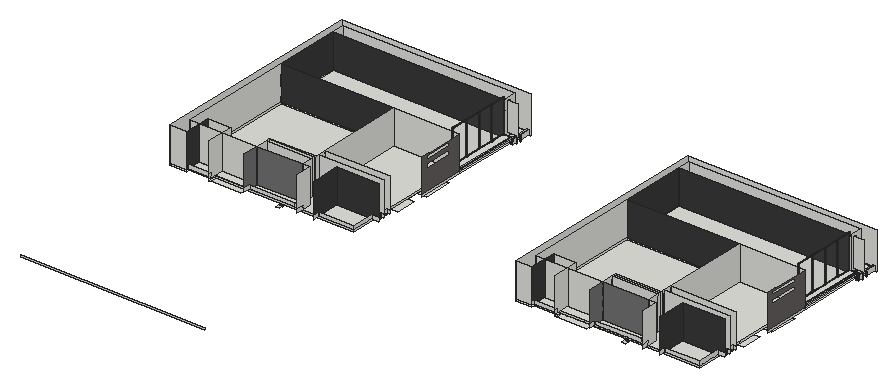
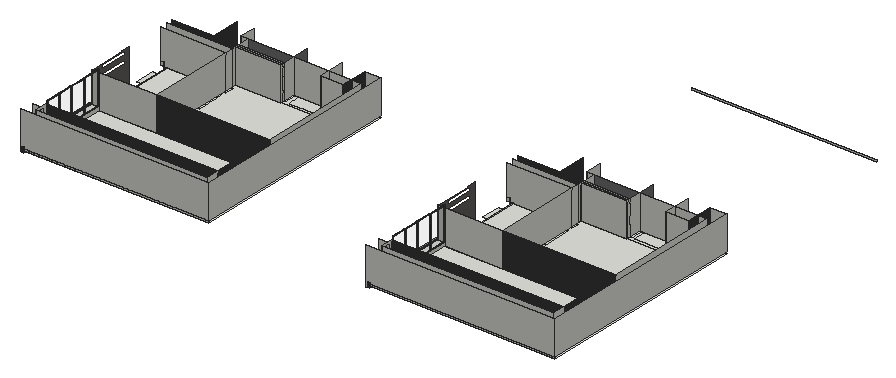
# SketchUp Ruby script. Lengths in inches.
U = 1.inch
M = Sketchup.active_model
def pt(a) = Geom::Point3d.new(a.map { |v| v * U })
def face(e, loops, mat)
  f = e.add_face(loops[0].map { |a| pt(a) })
  loops[1..].each { |l| e.add_face(l.map { |a| pt(a) }).erase! }
  f.material = f.back_material = mat if mat
  f
end
# faces: each face lists its corners as indices into pts; further lists are holes
def faces(e, pts, list, mat = nil) = list.each { |f| face(e, (f[0].is_a?(Array) ? f : [f]).map { |l| l.map { |i| pts[i] } }, mat) }
# xy, xz, yz: faces in a plane at the given z, y or x. An outline is a flat list of corners, or four numbers for a rectangle; further outlines are holes
def ring(l) = l.size == 4 ? [[l[0], l[1]], [l[2], l[1]], [l[2], l[3]], [l[0], l[3]]] : l.each_slice(2).to_a
def flat(e, list, mat, &to3) = list.each { |f| face(e, (f[0].is_a?(Array) ? f : [f]).map { |l| ring(l).map { |u, v| to3.(u, v) } }, mat) }
def xy(e, z, list, mat = nil) = flat(e, list, mat) { |x, y| [x, y, z] }
def xz(e, y, list, mat = nil) = flat(e, list, mat) { |x, z| [x, y, z] }
def yz(e, x, list, mat = nil) = flat(e, list, mat) { |y, z| [x, y, z] }
def lines(e, pts, list) = list.each { |a, b| e.add_line(pt(pts[a]), pt(pts[b])) }
# prism: a flat outline (further loops are holes) pulled along v
def prism(e, loops, v, mat = nil)
  f = face(e, loops, mat); d = Geom::Vector3d.new(v.map { |x| x * U })
  f.pushpull(f.normal.samedirection?(d) ? d.length : -d.length)
end
def box(e, o, s, mat = nil) = prism(e, [[o, [o[0] + s[0], o[1], o[2]], [o[0] + s[0], o[1] + s[1], o[2]], [o[0], o[1] + s[1], o[2]]]], [0, 0, s[2]], mat)
def at(x, y, z, deg = 0) = Geom::Transformation.translation(pt([x, y, z])) * Geom::Transformation.rotation(ORIGIN, Z_AXIS, deg.degrees)
def axes(o, x, y, z) = Geom::Transformation.new([*x, 0, *y, 0, *z, 0, *pt(o).to_a, 1])
def part(name) = M.definitions.add(name)
# library, detail: a bought-in or finely detailed component or shape, given as its bounding box
def library(name, o, s) = part(name).tap { |d| box(d.entities, o, s) }
def detail(e, o, s) = box(e.add_group.entities, o, s)
def put(e, d, t, mat = nil) = e.add_instance(d, t).tap { |i| i.material = mat if mat }
def group(e, t, mat = nil) = e.add_group.tap { |g| g.transformation = t; g.material = mat if mat }.entities
root = M.entities
M.materials.add("Glazing").color = [128, 128, 128]
M.materials["Glazing"].alpha = 0.05
M.materials.add("Powdercoating").color = [41, 44, 40]
M.materials.add("[Color M05]").color = [114, 114, 114]
M.materials.add("[Color M07]").color = [58, 58, 58]
M.materials.add("[Concrete Tile]").color = [165, 155, 133]
M.materials.add("[Stone Marble]").color = [99, 95, 94]
c1 = part("Group\#15")
xy(c1.entities,0,[[0,-55.94,0.71,45.94]])
xy(c1.entities,0.2,[[0,-55.94,0.47,45.94],[0.47,45.94,0.71,46.42]])
xy(c1.entities,2.36,[[0.47,-55.94,0.71,46.42]])
xz(c1.entities,-55.94,[[0,0,0.71,0,0.71,2.36,0.47,2.36,0.47,0.2,0,0.2]])
xz(c1.entities,45.94,[[0,0,0.71,0.2]])
xz(c1.entities,46.42,[[0.47,0.2,0.71,2.36]])
yz(c1.entities,0,[[-55.94,0,45.94,0.2]])
yz(c1.entities,0.47,[[-55.94,0.2,46.42,2.36]])
yz(c1.entities,0.71,[[-55.94,0,45.94,0,45.94,0.2,46.42,0.2,46.42,2.36,-55.94,2.36]])
c2 = part("Group\#7")
xy(c2.entities,0,[[0,-59.09,0.71,45.94]])
xy(c2.entities,0.2,[[0,-59.09,0.47,45.94],[0.47,45.94,0.71,46.42]])
xy(c2.entities,2.36,[[0.47,-59.09,0.71,46.42]])
xz(c2.entities,-59.09,[[0,0,0.71,0,0.71,2.36,0.47,2.36,0.47,0.2,0,0.2]])
xz(c2.entities,45.94,[[0,0,0.71,0.2]])
xz(c2.entities,46.42,[[0.47,0.2,0.71,2.36]])
yz(c2.entities,0,[[-59.09,0,45.94,0.2]])
yz(c2.entities,0.47,[[-59.09,0.2,46.42,2.36]])
yz(c2.entities,0.71,[[-59.09,0,45.94,0,45.94,0.2,46.42,0.2,46.42,2.36,-59.09,2.36]])
c3 = part("Group\#16")
prism(c3.entities,[[[0.47,-56.18,0.2],[0,-56.18,0.2],[0,-56.18,0],[0.71,-56.18,0],[0.71,-56.18,2.36],[0.47,-56.18,2.36]]],[0,28.68,0])
c4 = part("Group\#10")
box(c4.entities,[-0.73,0,0],[27.99,0.55,102.05])
c5 = part("Group\#18")
xy(c5.entities,0,[[0.47,-56.18,0.47,-55.47,0,-55.47,0,-28.21,1.18,-28.21,1.18,-56.18]])
xy(c5.entities,0.2,[[0.71,-56.18,1.18,-28.21],[0,-55.47,0.47,-28.21],[0.47,-28.21,0.71,-27.74]])
xy(c5.entities,2.36,[[0.47,-56.18,0.71,-27.74]])
xz(c5.entities,-56.18,[[0.47,0,1.18,0,1.18,0.2,0.71,0.2,0.71,2.36,0.47,2.36]])
xz(c5.entities,-55.47,[[0,0,0.47,0.2]])
xz(c5.entities,-28.21,[[0,0,1.18,0.2]])
xz(c5.entities,-27.74,[[0.47,0.2,0.71,2.36]])
yz(c5.entities,0,[[-55.47,0,-28.21,0.2]])
yz(c5.entities,0.47,[[-56.18,0,-55.47,0.2],[-56.18,0.2,-27.74,2.36]])
yz(c5.entities,0.71,[[-56.18,0.2,-27.74,2.36]])
yz(c5.entities,1.18,[[-56.18,0,-28.21,0.2]])
c6 = part("Group\#34")
xy(c6.entities,0,[[-20.45,0,7.76,1.22]])
xy(c6.entities,0.06,[[-20.39,0.06,7.7,1.22]])
xy(c6.entities,0.47,[[-19.98,0,7.28,0.06]])
xy(c6.entities,101.89,[[-19.98,0,7.28,0.06]])
xy(c6.entities,102.3,[[-20.39,0.06,7.7,1.22]])
xy(c6.entities,102.36,[[-20.45,0,7.76,1.22]])
xz(c6.entities,0,[[[-20.45,0,7.76,102.36],[-19.98,0.47,7.28,101.89]]])
xz(c6.entities,0.06,[[[-20.39,0.06,7.7,102.3],[-19.98,0.47,7.28,101.89]]])
xz(c6.entities,1.22,[[[-20.45,0,7.76,102.36],[-20.39,0.06,7.7,102.3]]])
yz(c6.entities,-20.45,[[0,0,1.22,102.36]])
yz(c6.entities,-20.39,[[0.06,0.06,1.22,102.3]])
yz(c6.entities,-19.98,[[0,0.47,0.06,101.89]])
yz(c6.entities,7.28,[[0,0.47,0.06,101.89]])
yz(c6.entities,7.7,[[0.06,0.06,1.22,102.3]])
yz(c6.entities,7.76,[[0,0,1.22,102.36]])
c7 = part("Group\#6")
put(c7.entities,c1,axes([27.97,0,7.875],[1,0,0],[0,0,-1],[0,1,0]),"Powdercoating")
put(c7.entities,c2,axes([0.71,0,6.8],[-1,0,0],[0,0,-0.97687],[0,1,0]),"Powdercoating")
put(c7.entities,c3,axes([-27.5,0,-38.07],[0,0,-1],[-1,0,0],[0,1,0]),"Powdercoating")
put(c7.entities,c4,at(1.12,0.35,-38.39),"Glazing")
put(c7.entities,c5,axes([-27.5,0,63.35],[0,0,1],[-1,0,0],[0,1,0]),"Powdercoating")
put(c7.entities,c6,at(20.6875,1.0625,-38.54),"Powdercoating")
c8 = part("Sliding door assembly")
put(c8.entities,c7,at(-1.18,4.5,38.86))
g1 = group(c8.entities,at(84.74,4.5,38.86))
put(g1,c1,axes([-27.97,0,7.875],[-1,0,0],[0,0,-1],[0,1,0]),"Powdercoating")
put(g1,c2,axes([-0.71,0,6.8],[1,0,0],[0,0,-0.97687],[0,1,0]),"Powdercoating")
put(g1,c3,axes([27.5,0,-38.07],[0,0,-1],[1,0,0],[0,1,0]),"Powdercoating")
put(g1,c4,axes([-1.12,0.35,-38.39],[-1,0,0],[0,1,0],[0,0,1]),"Glazing")
put(g1,c5,axes([27.5,0,63.35],[0,0,1],[1,0,0],[0,1,0]),"Powdercoating")
put(g1,c6,axes([-20.6875,1.0625,-38.54],[-1,0,0],[0,1,0],[0,0,1]),"Powdercoating")
g2 = group(c8.entities,at(56.0625,4.5,38.86))
put(g2,c1,axes([-27.97,0,7.875],[-1,0,0],[0,0,-1],[0,1,0]),"Powdercoating")
put(g2,c3,axes([27.5,0,-38.07],[0,0,-1],[1,0,0],[0,1,0]),"Powdercoating")
put(g2,c4,axes([-1.12,0.35,-38.39],[-1,0,0],[0,1,0],[0,0,1]),"Glazing")
put(g2,c5,axes([27.5,0,63.35],[0,0,1],[1,0,0],[0,1,0]),"Powdercoating")
put(g2,c6,axes([-20.6875,1.0625,-38.54],[-1,0,0],[0,1,0],[0,0,1]),"Powdercoating")
g3 = group(g2,at(-0.71,0,6.8),"Powdercoating")
xy(g3,-45.34,[[0.47,0.2,0.71,2.36]])
xy(g3,-44.88,[[0,0,0.71,0.2]])
xy(g3,57.73,[[0,0,0.71,0,0.71,2.36,0.47,2.36,0.47,0.2,0,0.2]])
xz(g3,0,[[0,-44.88,0.71,57.73]])
xz(g3,0.2,[[0.47,-45.34,0.71,-44.88],[0,-44.88,0.47,57.73]])
xz(g3,2.36,[[0.47,-45.34,0.71,57.73]])
yz(g3,0,[[0,-44.88,0.2,57.73]])
yz(g3,0.47,[[0.2,-45.34,2.36,57.73]])
yz(g3,0.71,[[0.2,-45.34,2.36,-45.34,2.36,57.73,0,57.73,0,-44.88,0.2,-44.88]])
put(c8.entities,c7,axes([-33.94,4.5,38.86],[1.14218,0,0],[0,1,0],[0,0,1]))
c9 = part("sliding door")
put(c9.entities,c8,at(0,-4.5,-0.08))
xy(root,117.41,[[671.25,3528.25,913.875,3628.31],[1889.4375,3528.25,2132.0625,3628.31]])
xy(root,126,[[262.875,3214.625,262.875,3969.0625,913.875,3969.0625,913.875,3897.9,890.875,3897.9,890.875,3946.0625,285.875,3946.0625,285.875,3237.625,319.53,3237.625,319.53,3214.625],[399.88,3214.625,406.68,3237.625],[406.68,3214.625,511.23,3237.625],[634.11,3214.625,647.8,3229.61],[1481.0625,3214.625,1481.0625,3969.0625,2132.0625,3969.0625,2132.0625,3897.9,2109.0625,3897.9,2109.0625,3946.0625,1504.0625,3946.0625,1504.0625,3237.625,1537.72,3237.625,1537.72,3214.625],
  [1618.07,3214.625,1624.87,3237.625],[1624.87,3214.625,1729.42,3237.625],[1852.3,3214.625,1865.99,3229.61],[319.53,3226.125,399.88,3237.625],[1537.72,3226.125,1618.07,3237.625],
  [285.875,3237.625,319.53,3248.75],[319.53,3237.625,399.88,3248.75],[399.88,3237.625,406.68,3248.75],[406.68,3237.625,511.23,3248.75],[511.23,3237.625,521.59,3248.75],
  [521.59,3237.625,634.11,3248.75],[634.11,3237.625,709.87,3248.75],[709.87,3237.625,767.19,3248.75],[767.19,3237.625,817,3248.75],[817,3237.625,890.875,3248.75],
  [1504.0625,3237.625,1537.72,3248.75],[1537.72,3237.625,1618.07,3248.75],[1618.07,3237.625,1624.87,3248.75],[1624.87,3237.625,1729.42,3248.75],[1729.42,3237.625,1739.78,3248.75],
  [1739.78,3237.625,1852.3,3248.75],[1852.3,3237.625,1928.05,3248.75],[1928.05,3237.625,1985.38,3248.75],[1985.38,3237.625,2035.1875,3248.75],[2035.1875,3237.625,2109.0625,3248.75],
  [285.875,3248.75,319.53,3248.75,319.53,3307.9375,399.88,3307.9375,399.88,3248.75,406.68,3248.75,406.68,3307.9375,511.23,3307.9375,511.23,3248.75,521.59,3248.75,521.59,3307.9375,709.87,3307.9375,709.87,3248.75,767.19,3248.75,767.19,3317.34,285.875,3317.34],[319.53,3248.75,399.88,3307.9375],[406.68,3248.75,511.23,3307.9375],[521.59,3248.75,634.11,3307.9375],[634.11,3248.75,709.87,3307.9375],
  [767.19,3248.75,817,3317.34],[817,3248.75,890.875,3317.34],[1504.0625,3248.75,1537.72,3248.75,1537.72,3307.9375,1618.07,3307.9375,1618.07,3248.75,1624.87,3248.75,1624.87,3307.9375,1729.42,3307.9375,1729.42,3248.75,1739.78,3248.75,1739.78,3307.9375,1928.05,3307.9375,1928.05,3248.75,1985.38,3248.75,1985.38,3317.34,1504.0625,3317.34],[1537.72,3248.75,1618.07,3307.9375],[1624.87,3248.75,1729.42,3307.9375],
  [1739.78,3248.75,1852.3,3307.9375],[1852.3,3248.75,1928.05,3307.9375],[1985.38,3248.75,2035.1875,3317.34],[2035.1875,3248.75,2109.0625,3317.34],[285.875,3317.34,817,3317.34,817,3340.76,683.6875,3340.76,683.6875,3368.39,817,3368.39,817,3385.6,683.6875,3385.6,683.6875,3484.97,890.875,3484.97,890.875,3672.5,285.875,3672.5],
  [817,3317.34,890.875,3340.76],[1504.0625,3317.34,2035.1875,3317.34,2035.1875,3340.76,1901.875,3340.76,1901.875,3368.39,2035.1875,3368.39,2035.1875,3385.6,1901.875,3385.6,1901.875,3484.97,2109.0625,3484.97,2109.0625,3672.5,1504.0625,3672.5],[2035.1875,3317.34,2109.0625,3340.76],[683.6875,3340.76,817,3368.39],[817,3340.76,890.875,3368.39],
  [890.875,3340.76,902.375,3368.39],[1901.875,3340.76,2035.1875,3368.39],[2035.1875,3340.76,2109.0625,3368.39],[2109.0625,3340.76,2120.5625,3368.39],[817,3368.39,890.875,3385.6],
  [2035.1875,3368.39,2109.0625,3385.6],[683.6875,3385.6,890.875,3484.97],[1901.875,3385.6,2109.0625,3484.97],[890.875,3402.54,913.875,3473.84],[2109.0625,3402.54,2132.0625,3473.84],
  [285.875,3672.5,890.875,3900.52],[890.875,3672.5,913.875,3897.9],[1504.0625,3672.5,2109.0625,3900.52],[2109.0625,3672.5,2132.0625,3897.9]])
xy(root,132,[[262.875,3214.625,262.875,3969.0625,913.875,3969.0625,913.875,3897.9,890.875,3897.9,890.875,3946.0625,285.875,3946.0625,285.875,3237.625,319.53,3237.625,319.53,3214.625],[1481.0625,3214.625,1481.0625,3969.0625,2132.0625,3969.0625,2132.0625,3897.9,2109.0625,3897.9,2109.0625,3946.0625,1504.0625,3946.0625,1504.0625,3237.625,1537.72,3237.625,1537.72,3214.625],[319.53,3222.3125,399.88,3237.625],[1537.72,3222.3125,1618.07,3237.625],[285.875,3237.625,319.53,3270.4375],
  [319.53,3237.625,399.88,3270.4375],[399.88,3237.625,523.04,3270.4375],[523.04,3237.625,683.6875,3270.4375],[683.6875,3237.625,709.87,3270.4375],[709.87,3237.625,709.87,3270.4375,683.6875,3270.4375,683.6875,3340.76,890.875,3340.76,890.875,3317.34,767.19,3317.34,767.19,3237.625],
  [767.19,3237.625,890.875,3317.34],[1504.0625,3237.625,1537.72,3270.4375],[1537.72,3237.625,1618.07,3270.4375],[1618.07,3237.625,1741.23,3270.4375],[1741.23,3237.625,1901.875,3270.4375],
  [1901.875,3237.625,1928.05,3270.4375],[1928.05,3237.625,1928.05,3270.4375,1901.875,3270.4375,1901.875,3340.76,2109.0625,3340.76,2109.0625,3317.34,1985.38,3317.34,1985.38,3237.625],[1985.38,3237.625,2109.0625,3317.34],[319.53,3270.4375,399.88,3307.9375],[523.04,3270.4375,683.6875,3312.25],
  [1537.72,3270.4375,1618.07,3307.9375],[1741.23,3270.4375,1901.875,3312.25],[523.04,3312.25,683.6875,3321.375],[1741.23,3312.25,1901.875,3321.375],[523.04,3321.375,683.6875,3328.125],
  [1741.23,3321.375,1901.875,3328.125],[683.6875,3340.76,890.875,3368.39],[890.875,3340.76,902.375,3368.39],[1901.875,3340.76,2109.0625,3368.39],[2109.0625,3340.76,2120.5625,3368.39],
  [683.6875,3368.39,890.875,3672.87],[1901.875,3368.39,2109.0625,3672.87],[285.875,3672.87,886.75,3672.87,886.75,3897.9,890.875,3897.9,890.875,3901.51,285.875,3901.51],[886.75,3672.87,890.875,3897.9],[890.875,3672.87,913.875,3897.9],
  [1504.0625,3672.87,2104.9375,3672.87,2104.9375,3897.9,2109.0625,3897.9,2109.0625,3901.51,1504.0625,3901.51],[2104.9375,3672.87,2109.0625,3897.9],[2109.0625,3672.87,2132.0625,3897.9]])
xy(root,143.875,[[913.875,3672.5,921.125,3672.87],[2132.0625,3672.5,2139.3125,3672.87],[886.75,3672.87,913.875,3897.9],[913.875,3672.87,921.125,3897.9],[2104.9375,3672.87,2132.0625,3897.9],
  [2132.0625,3672.87,2139.3125,3897.9],[913.875,3897.9,921.125,3901.51],[2132.0625,3897.9,2139.3125,3901.51]])
xy(root,144.25,[[913.875,3672.5,921.125,3672.87],[2132.0625,3672.5,2139.3125,3672.87]])
xz(root,2554.375,[[262.875,126,913.875,132]])
xz(root,3214.625,[[262.875,132,319.53,252],[1481.0625,132,1537.72,252]])
xz(root,3214.625,[[521.59,132,523.04,252],[1739.78,132,1741.23,252]],"[Concrete Tile]")
xz(root,3222.3125,[[319.53,132,399.88,145.375],[1537.72,132,1618.07,145.375]])
xz(root,3229.61,[[634.11,124.32,647.8,126],[1852.3,124.32,1865.99,126]])
xz(root,3237.625,[[285.875,126,890.875,132],[1504.0625,126,2109.0625,132],[523.04,132,683.6875,145.375],[683.6875,132,709.87,145.375],[767.19,132,890.875,145.375],
  [1741.23,132,1901.875,145.375],[1901.875,132,1928.05,145.375],[1985.38,132,2109.0625,145.375]])
xz(root,3270.4375,[[285.875,132,523.04,252],[683.6875,132,709.87,252],[1504.0625,132,1741.23,252],[1901.875,132,1928.05,252]])
xz(root,3270.4375,[[523.04,132,683.6875,252],[1741.23,132,1901.875,252]],"[Color M05]")
xz(root,3307.9375,[[319.53,132,399.88,252],[1537.72,132,1618.07,252]])
xz(root,3312.25,[[523.04,132,683.6875,252],[1741.23,132,1901.875,252]])
xz(root,3317.34,[[890.875,132,913.875,145.375],[2109.0625,132,2132.0625,145.375]])
xz(root,3317.34,[[767.19,132,890.875,132,890.875,147.125,913.875,147.125,913.875,252,767.19,252],[1985.38,132,2109.0625,132,2109.0625,147.125,2132.0625,147.125,2132.0625,252,1985.38,252]],"[Color M07]")
xz(root,3321.375,[[523.04,132,683.6875,252],[1741.23,132,1901.875,252]])
xz(root,3328.125,[[523.04,132,683.6875,252],[1741.23,132,1901.875,252]])
xz(root,3340.76,[[683.6875,132,683.6875,252,913.875,252,913.875,145.375,902.375,145.375,902.375,132],[902.375,132,913.875,145.375],[1901.875,132,1901.875,252,2132.0625,252,2132.0625,145.375,2120.5625,145.375,2120.5625,132],[2120.5625,132,2132.0625,145.375]])
xz(root,3368.39,[[683.6875,132,902.375,132,902.375,145.375,913.875,145.375,913.875,252,683.6875,252],[902.375,132,913.875,145.375],[1901.875,132,2120.5625,132,2120.5625,145.375,2132.0625,145.375,2132.0625,252,1901.875,252],[2120.5625,132,2132.0625,145.375]])
xz(root,3672.5,[[913.875,143.875,921.125,144.25],[2132.0625,143.875,2139.3125,144.25]])
xz(root,3672.87,[[683.6875,132,683.6875,252,913.875,252,913.875,143.875,886.75,143.875,886.75,132],[886.75,132,913.875,143.875],[1901.875,132,1901.875,252,2132.0625,252,2132.0625,143.875,2104.9375,143.875,2104.9375,132],[2104.9375,132,2132.0625,143.875],[913.875,143.875,921.125,144.25],
  [2132.0625,143.875,2139.3125,144.25],[913.875,144.25,921.125,145.375],[2132.0625,144.25,2139.3125,145.375]])
xz(root,3672.87,[[285.875,132,683.6875,252],[1504.0625,132,1901.875,252]],"[Color M07]")
xz(root,3897.9,[[886.75,132,890.875,136.875],[2104.9375,132,2109.0625,136.875],[886.75,136.875,890.875,143.875],[2104.9375,136.875,2109.0625,143.875],[913.875,143.875,921.125,145.375],
  [2132.0625,143.875,2139.3125,145.375]])
xz(root,3897.9,[[890.875,132,913.875,136.875],[2109.0625,132,2132.0625,136.875],[890.875,136.875,913.875,143.875],[2109.0625,136.875,2132.0625,143.875]],"[Color M07]")
xz(root,3901.51,[[913.875,120.4375,921.125,136.875],[2132.0625,120.4375,2139.3125,136.875],[913.875,136.875,921.125,143.875],[2132.0625,136.875,2139.3125,143.875]])
xz(root,3901.51,[[285.875,132,890.875,252],[1504.0625,132,2109.0625,252]],"[Color M07]")
xz(root,3912.16,[[921.125,120.4375,927.0625,136.875],[2139.3125,120.4375,2145.25,136.875],[927.0625,143.875,927.0625,145.375,890.875,145.375,890.875,245.15,927.75,245.15,927.75,143.875],[2145.25,143.875,2145.25,145.375,2109.0625,145.375,2109.0625,245.15,2145.9375,245.15,2145.9375,143.875]])
xz(root,3929.52,[[921.125,120.4375,927.0625,136.875],[2139.3125,120.4375,2145.25,136.875]])
xz(root,3946.0625,[[285.875,126,890.875,132],[1504.0625,126,2109.0625,132],[285.875,132,890.875,252],[1504.0625,132,2109.0625,252]])
xz(root,3969.0625,[[921.125,120.4375,921.125,136.875,913.875,136.875,913.875,132,262.875,132,262.875,252,927.75,252,927.75,120.4375],[913.875,120.4375,921.125,136.875],[2139.3125,120.4375,2139.3125,136.875,2132.0625,136.875,2132.0625,132,1481.0625,132,1481.0625,252,2145.9375,252,2145.9375,120.4375],[2132.0625,120.4375,2139.3125,136.875],[262.875,126,913.875,132],
  [1481.0625,126,2132.0625,132]])
yz(root,262.875,[[3214.625,132,3969.0625,252]])
yz(root,285.875,[[3237.625,126,3946.0625,132],[3270.4375,132,3672.87,252],[3901.51,132,3946.0625,252]])
yz(root,285.875,[[3672.87,132,3901.51,252]],"[Color M07]")
yz(root,319.53,[[3214.625,132,3222.3125,145.375]])
yz(root,319.53,[[3222.3125,132,3307.9375,132,3307.9375,252,3214.625,252,3214.625,145.375,3222.3125,145.375]],"[Color M07]")
yz(root,399.88,[[3214.625,132,3222.3125,145.375],[3222.3125,132,3222.3125,145.375,3214.625,145.375,3214.625,252,3307.9375,252,3307.9375,132]])
yz(root,523.04,[[3214.625,132,3237.625,145.375],[3270.4375,132,3312.25,252],[3312.25,132,3321.375,252],[3321.375,132,3328.125,252]])
yz(root,523.04,[[3237.625,132,3270.4375,132,3270.4375,252,3214.625,252,3214.625,145.375,3237.625,145.375]],"[Color M05]")
yz(root,683.6875,[[3270.4375,132,3312.25,252],[3312.25,132,3321.375,252],[3321.375,132,3328.125,252],[3328.125,132,3340.76,252],[3340.76,132,3368.39,252],
  [3368.39,132,3672.87,252]])
yz(root,709.87,[[3214.625,132,3237.625,145.375],[3237.625,132,3237.625,145.375,3214.625,145.375,3214.625,252,3270.4375,252,3270.4375,132]])
yz(root,767.19,[[3214.625,132,3237.625,145.375]])
yz(root,767.19,[[3237.625,132,3317.34,132,3317.34,252,3214.625,252,3214.625,147.125,3237.625,147.125]],"[Color M07]")
yz(root,886.75,[[3672.87,132,3897.9,143.875]])
yz(root,890.875,[[3237.625,126,3946.0625,132],[3237.625,132,3317.34,145.375],[3897.9,132,3901.51,252],[[3901.51,132,3946.0625,252],[3912.16,145.375,3929.52,245.15]]])
yz(root,902.375,[[3340.76,132,3368.39,145.375]])
yz(root,913.875,[[3897.9,120.4375,3901.51,126],[3901.51,120.4375,3969.0625,126],[3508.34,126,3672.5,132],[3901.51,126,3969.0625,132],[3672.5,132,3672.87,143.875],
  [3672.87,132,3897.9,143.875],[3897.9,132,3901.51,136.875],[3901.51,132,3969.0625,136.875],[3897.9,136.875,3901.51,143.875],[3672.5,143.875,3672.87,144.25],
  [3672.87,143.875,3897.9,145.375]])
yz(root,913.875,[[[3508.34,132,3672.5,132,3672.5,144.25,3672.87,144.25,3672.87,248.9375,3539.2,248.9375,3539.2,252,3508.34,252],[3528.25,206.6875,3628.31,220.18],[3528.25,234.11,3628.31,246.61]]],"[Stone Marble]")
yz(root,921.125,[[3898.89,120.4375,3901.51,136.875],[3901.51,120.4375,3912.16,136.875],[3929.52,120.4375,3969.0625,136.875],[3898.89,136.875,3901.51,143.875],[3672.5,143.875,3672.87,144.25],
  [3672.87,143.875,3897.9,145.375]])
yz(root,1481.0625,[[3214.625,132,3969.0625,252]])
yz(root,1504.0625,[[3237.625,126,3946.0625,132],[3270.4375,132,3672.87,252],[3901.51,132,3946.0625,252]])
yz(root,1504.0625,[[3672.87,132,3901.51,252]],"[Color M07]")
yz(root,1537.72,[[3214.625,132,3222.3125,145.375]])
yz(root,1537.72,[[3222.3125,132,3307.9375,132,3307.9375,252,3214.625,252,3214.625,145.375,3222.3125,145.375]],"[Color M07]")
yz(root,1618.07,[[3214.625,132,3222.3125,145.375],[3222.3125,132,3222.3125,145.375,3214.625,145.375,3214.625,252,3307.9375,252,3307.9375,132]])
yz(root,1741.23,[[3214.625,132,3237.625,145.375],[3270.4375,132,3312.25,252],[3312.25,132,3321.375,252],[3321.375,132,3328.125,252]])
yz(root,1741.23,[[3237.625,132,3270.4375,132,3270.4375,252,3214.625,252,3214.625,145.375,3237.625,145.375]],"[Color M05]")
yz(root,1901.875,[[3270.4375,132,3312.25,252],[3312.25,132,3321.375,252],[3321.375,132,3328.125,252],[3328.125,132,3340.76,252],[3340.76,132,3368.39,252],
  [3368.39,132,3672.87,252]])
yz(root,1928.05,[[3214.625,132,3237.625,145.375],[3237.625,132,3237.625,145.375,3214.625,145.375,3214.625,252,3270.4375,252,3270.4375,132]])
yz(root,1985.38,[[3214.625,132,3237.625,145.375]])
yz(root,1985.38,[[3237.625,132,3317.34,132,3317.34,252,3214.625,252,3214.625,147.125,3237.625,147.125]],"[Color M07]")
yz(root,2104.9375,[[3672.87,132,3897.9,143.875]])
yz(root,2109.0625,[[3237.625,126,3946.0625,132],[3237.625,132,3317.34,145.375],[3897.9,132,3901.51,252],[[3901.51,132,3946.0625,252],[3912.16,145.375,3929.52,245.15]]])
yz(root,2120.5625,[[3340.76,132,3368.39,145.375]])
yz(root,2132.0625,[[3897.9,120.4375,3901.51,126],[3901.51,120.4375,3969.0625,126],[3508.34,126,3672.5,132],[3901.51,126,3969.0625,132],[3672.5,132,3672.87,143.875],
  [3672.87,132,3897.9,143.875],[3897.9,132,3901.51,136.875],[3901.51,132,3969.0625,136.875],[3897.9,136.875,3901.51,143.875],[3672.5,143.875,3672.87,144.25],
  [3672.87,143.875,3897.9,145.375]])
yz(root,2132.0625,[[[3508.34,132,3672.5,132,3672.5,144.25,3672.87,144.25,3672.87,248.9375,3539.2,248.9375,3539.2,252,3508.34,252],[3528.25,206.6875,3628.31,220.18],[3528.25,234.11,3628.31,246.61]]],"[Stone Marble]")
yz(root,2139.3125,[[3898.89,120.4375,3901.51,136.875],[3901.51,120.4375,3912.16,136.875],[3929.52,120.4375,3969.0625,136.875],[3898.89,136.875,3901.51,143.875],[3672.5,143.875,3672.87,144.25],
  [3672.87,143.875,3897.9,145.375]])
p = [[2132.0625,3900.52,120.4375],[2139.3125,3900.52,120.4375],[913.875,3900.52,120.4375],[921.125,3900.52,120.4375]]
lines(root,p,[[0,1],[2,3]])
put(root,c9,axes([2109.0625,3737.91,143.875],[0,1.90384,0],[-1,0,0],[0,0,1.13691]),"[Color M07]")
put(root,c9,axes([890.875,3737.91,143.875],[0,1.90384,0],[-1,0,0],[0,0,1.13691]),"[Color M07]")
